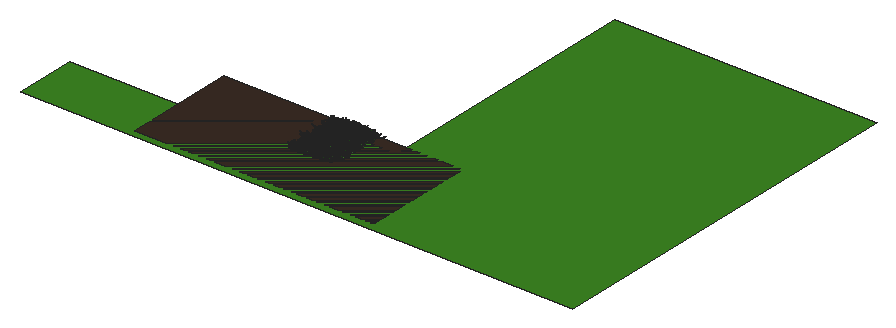
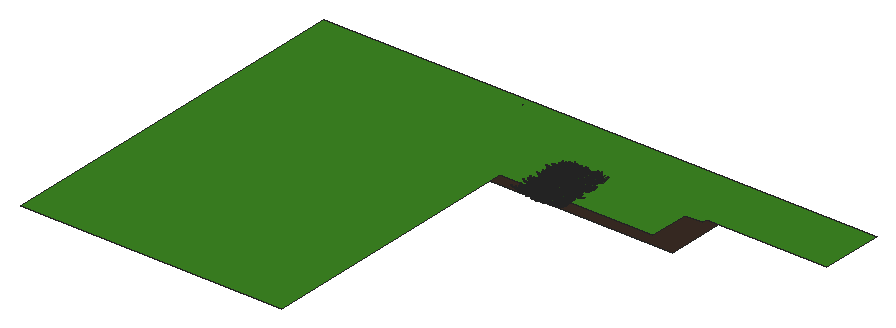
# SketchUp Ruby script. Lengths in inches.
U = 1.inch
M = Sketchup.active_model
def pt(a) = Geom::Point3d.new(a.map { |v| v * U })
def face(e, loops, mat)
  f = e.add_face(loops[0].map { |a| pt(a) })
  loops[1..].each { |l| e.add_face(l.map { |a| pt(a) }).erase! }
  f.material = f.back_material = mat if mat
  f
end
# faces: each face lists its corners as indices into pts; further lists are holes
def faces(e, pts, list, mat = nil) = list.each { |f| face(e, (f[0].is_a?(Array) ? f : [f]).map { |l| l.map { |i| pts[i] } }, mat) }
# xy, xz, yz: faces in a plane at the given z, y or x. An outline is a flat list of corners, or four numbers for a rectangle; further outlines are holes
def ring(l) = l.size == 4 ? [[l[0], l[1]], [l[2], l[1]], [l[2], l[3]], [l[0], l[3]]] : l.each_slice(2).to_a
def flat(e, list, mat, &to3) = list.each { |f| face(e, (f[0].is_a?(Array) ? f : [f]).map { |l| ring(l).map { |u, v| to3.(u, v) } }, mat) }
def xy(e, z, list, mat = nil) = flat(e, list, mat) { |x, y| [x, y, z] }
def xz(e, y, list, mat = nil) = flat(e, list, mat) { |x, z| [x, y, z] }
def yz(e, x, list, mat = nil) = flat(e, list, mat) { |y, z| [x, y, z] }
def lines(e, pts, list) = list.each { |a, b| e.add_line(pt(pts[a]), pt(pts[b])) }
# prism: a flat outline (further loops are holes) pulled along v
def prism(e, loops, v, mat = nil)
  f = face(e, loops, mat); d = Geom::Vector3d.new(v.map { |x| x * U })
  f.pushpull(f.normal.samedirection?(d) ? d.length : -d.length)
end
def box(e, o, s, mat = nil) = prism(e, [[o, [o[0] + s[0], o[1], o[2]], [o[0] + s[0], o[1] + s[1], o[2]], [o[0], o[1] + s[1], o[2]]]], [0, 0, s[2]], mat)
def at(x, y, z, deg = 0) = Geom::Transformation.translation(pt([x, y, z])) * Geom::Transformation.rotation(ORIGIN, Z_AXIS, deg.degrees)
def axes(o, x, y, z) = Geom::Transformation.new([*x, 0, *y, 0, *z, 0, *pt(o).to_a, 1])
def part(name) = M.definitions.add(name)
# library, detail: a bought-in or finely detailed component or shape, given as its bounding box
def library(name, o, s) = part(name).tap { |d| box(d.entities, o, s) }
def detail(e, o, s) = box(e.add_group.entities, o, s)
def put(e, d, t, mat = nil) = e.add_instance(d, t).tap { |i| i.material = mat if mat }
def group(e, t, mat = nil) = e.add_group.tap { |g| g.transformation = t; g.material = mat if mat }.entities
root = M.entities
M.materials.add("Material82").color = [68, 110, 58]
M.materials.add("Material83").color = [48, 90, 38]
M.materials.add("Material84").color = [68, 110, 48]
M.materials.add("Material85").color = [48, 90, 48]
M.materials.add("Material86").color = [58, 110, 58]
M.materials.add("Material87").color = [58, 90, 38]
M.materials.add("Material88").color = [68, 100, 58]
M.materials.add("Material89").color = [48, 100, 38]
M.materials.add("[Color M01]").color = [60, 133, 34]
M.materials.add("top-soil").color = [58, 44, 36]
c1 = part("grass00")
p = [[-0.6875,0.15,0],[-0.56,0.08,5.52],[-0.04,0.03,2.76],[0.48,-0.02,0],[0.35,-0.02,5.52],[-0.1,-0.14,5.52],
  [-0.12,0.65,8.37],[-0.42,0.65,8.37]]
faces(c1.entities,p,[[0,1,2,3],[3,2,4],[1,5,2],[5,4,2],[1,6,5],[4,5,6],[7,6,1]])
c2 = part("Group16\#1")
put(c2.entities,c1,axes([1.44,-0.61,-0.01],[0.05352,0.12609,0],[-0.10704,0.04543,0.07239],[0.06664,-0.02828,0.11628]),"Material85")
put(c2.entities,c1,axes([0.76,-0.15,-0.01],[0.04676,0.24062,0],[-0.23162,0.04501,0.06642],[0.0652,-0.01267,0.23595]),"Material82")
put(c2.entities,c1,axes([0.79,0.01,-0.01],[-0.00606,0.34651,0],[-0.34381,-0.00602,0.0432],[0.04319,0.00076,0.34386]))
put(c2.entities,c1,axes([1,0.23,-0.01],[-0.07192,0.31144,0],[-0.28722,-0.06632,0.1236],[0.12043,0.02781,0.29478]),"Material84")
put(c2.entities,c1,axes([1.66,0.77,-0.01],[-0.13828,0.29651,0],[-0.21551,-0.1005,0.22471],[0.20365,0.09498,0.23779]),"Material89")
put(c2.entities,c1,axes([0.6875,0.52,-0.01],[-0.18126,0.24051,0],[-0.22746,-0.17142,0.09788],[0.07817,0.05891,0.28481]),"Material84")
put(c2.entities,c1,axes([0.68,0.78,-0.01],[-0.215,0.18688,0],[-0.12385,-0.14248,0.21334],[0.13995,0.16101,0.18878]),"Material82")
put(c2.entities,c1,axes([0.56,1,-0.01],[-0.13756,0.07624,0],[-0.06159,-0.11112,0.0927],[0.04494,0.08108,0.12705]),"Material84")
put(c2.entities,c1,axes([0.2,0.64,-0.01],[-0.23729,0.07254,0],[-0.05711,-0.18681,0.153],[0.04473,0.14632,0.19535]),"Material89")
put(c2.entities,c1,axes([0.0625,0.72,-0.01],[-0.28874,0.02525,0],[-0.02179,-0.24916,0.14647],[0.01276,0.14591,0.25012]),"Material82")
put(c2.entities,c1,axes([-0.08,0.62,-0.01],[-0.34089,-0.04187,0],[0.03255,-0.26504,0.216],[-0.02633,0.21439,0.26703]),"Material89")
put(c2.entities,c1,axes([-0.34,0.98,-0.01],[-0.14314,-0.0493,0],[0.04397,-0.12769,0.06843],[-0.02228,0.0647,0.13505]),"Material89")
put(c2.entities,c1,axes([-0.87,1.45,-0.01],[-0.23488,-0.14114,0],[0.13761,-0.22901,0.06087],[-0.03135,0.05217,0.26717]))
put(c2.entities,c1,axes([-0.72,0.77,-0.01],[-0.14208,-0.13251,0],[0.07209,-0.0773,0.16301],[-0.11118,0.11922,0.1057]),"Material89")
put(c2.entities,c1,axes([-0.62,0.43,-0.01],[-0.14845,-0.21203,0],[0.18654,-0.13061,0.12304],[-0.10079,0.07057,0.22772]),"Material82")
put(c2.entities,c1,axes([-0.68,0.29,-0.01],[-0.13639,-0.32136,0],[0.31723,-0.13464,0.05579],[-0.05136,0.0218,0.34462]),"Material83")
put(c2.entities,c1,axes([-0.64,0.125,-0.01],[-0.0458,-0.23569,0],[0.22124,-0.043,0.08276],[-0.08124,0.01579,0.22538]),"Material86")
put(c2.entities,c1,axes([-1.6,-0.03,-0.01],[0.00576,-0.32897,0],[0.27526,0.00482,0.18018],[-0.18015,-0.00315,0.2753]),"Material84")
put(c2.entities,c1,axes([-1.36,-0.31,-0.01],[0.05718,-0.24765,0],[0.18172,0.04196,0.17267],[-0.16825,-0.03885,0.1865]),"Material89")
put(c2.entities,c1,axes([-1.54,-0.72,-0.01],[0.06537,-0.14017,0],[0.13555,0.06321,0.03939],[-0.0357,-0.01665,0.14956]))
put(c2.entities,c1,axes([-1.19,-0.9,-0.01],[0.09597,-0.12735,0],[0.11214,0.08451,0.07557],[-0.06035,-0.04548,0.14042]),"Material88")
put(c2.entities,c1,axes([-0.47,-0.54,-0.01],[0.11588,-0.10072,0],[0.0618,0.0711,0.12124],[-0.07953,-0.0915,0.0942]))
put(c2.entities,c1,axes([-0.47,-0.84,-0.01],[0.11927,-0.0661,0],[0.06603,0.11913,0.00646],[-0.00313,-0.00565,0.13621]),"Material84")
put(c2.entities,c1,axes([-0.38,-1.24,-0.01],[0.28037,-0.08571,0],[0.0618,0.20215,0.20315],[-0.05939,-0.19428,0.21139]),"Material88")
put(c2.entities,c1,axes([-0.06,-0.66,-0.01],[0.22719,-0.01987,0],[0.01247,0.14255,0.17758],[-0.01547,-0.17691,0.1431]),"Material87")
put(c2.entities,c1,axes([0.11,-0.89,-0.01],[0.14882,0.01828,0],[-0.01058,0.08611,0.12229],[0.01491,-0.12138,0.08676]),"Material85")
put(c2.entities,c1,axes([0.25,-0.72,-0.01],[0.20481,0.07053,0],[-0.06206,0.18022,0.10291],[0.03351,-0.0973,0.1906]),"Material85")
put(c2.entities,c1,axes([0.85,-1.42,-0.01],[0.16481,0.09904,0],[-0.09472,0.15762,0.05616],[0.02893,-0.04814,0.18389]),"Material84")
put(c2.entities,c1,axes([1.01,-1.09,-0.01],[0.21858,0.20385,0],[-0.17495,0.1876,0.15339],[0.10462,-0.11218,0.25652]),"Material89")
put(c2.entities,c1,axes([1.01,-0.71,-0.01],[0.08733,0.12473,0],[-0.06445,0.04512,0.13037],[0.1068,-0.07477,0.07867]),"Material85")
c3 = part("Group15\#1")
put(c3.entities,c2,at(0,0,0))
c4 = part("3darcstudiotree_grass00\#1")
put(c4.entities,c3,at(0,0,0))
xy(root,-29.74,[[1534.38,932.5,2096.625,932.5,2096.625,1318.18,1830.75,1318.18,1830.75,1040.81,1674.65,1040.81,1674.65,1000.12,1657.0625,1000.12,1657.0625,994.94,1534.38,994.94]],"[Color M01]")
xy(root,-29.74,[[1644.58,940.12,1887.61,1053.55]],"top-soil")
put(root,c4,axes([1764.68,1016.65,-29.74],[4.10776,0.45174,0],[-0.96091,1.35899,-0.03867],[-0.06802,0.0962,1.75619]))
put(root,c4,axes([1765.02,1044.86,-29.74],[0.30119,1.56993,0],[-3.74927,0.11187,-0.04286],[-0.21599,0.00644,1.42447]))
put(root,c4,axes([1766.64,1014.64,-29.74],[-3.02492,-1.16677,0],[2.80082,-1.12934,-0.0483],[0.17838,-0.07192,1.58573]))
put(root,c4,axes([1765.85,1046.92,-29.74],[3.50639,-1.07574,0],[2.8139,1.42651,-0.05588],[0.16686,0.08459,1.67045]))
put(root,c4,axes([1765.35,996.91,-29.74],[-0.3994,1.69229,0],[-4.36532,-0.16024,-0.02425],[-0.12976,-0.00476,1.76617]))
put(root,c4,axes([1767.22,1050.84,-29.74],[-0.91614,-1.55858,0],[4.47177,-0.40881,-0.01344],[0.0544,-0.00497,1.42931]))
put(root,c4,axes([1766.54,1031.09,-29.74],[-3.80907,0.85988,0],[-1.7501,-1.20575,-0.03218],[-0.10036,-0.06914,1.65786]))
put(root,c4,axes([1767.08,1001.97,-29.74],[1.67083,-1.60234,0],[3.7829,0.6135,-0.00107],[0.00454,0.00074,1.41133]))
put(root,c4,axes([1766.38,1049.21,-29.74],[-1.98309,1.36521,0],[-3.29696,-0.74485,-0.00674],[-0.03007,-0.00679,1.46389]))
put(root,c4,axes([1766.67,1011.9,-29.74],[-1.6341,1.38385,0],[-3.29524,-0.60518,-0.01596],[-0.09907,-0.01819,1.86544]))
put(root,c4,axes([1766.9,1017.96,-29.74],[-1.88391,1.25543,0],[-3.77395,-0.8808,-0.04665],[-0.1806,-0.04215,1.47851]))
put(root,c4,axes([1767.98,1041.09,-29.74],[-3.20908,-0.65771,0],[1.52004,-1.1535,-0.02241],[0.0705,-0.0535,1.68548]))
put(root,c4,axes([1767.1,1030.31,-29.74],[2.49471,1.02577,0],[-2.71621,1.02741,-0.02632],[-0.13149,0.04974,1.95302]))
put(root,c4,axes([1767.45,1037.94,-29.74],[4.09109,-0.59758,0],[1.20224,1.2801,-0.03178],[0.07676,0.08173,1.80429]))
put(root,c4,axes([1767.26,1005.53,-29.74],[2.32026,0.93484,0],[-2.86948,1.10768,-0.01876],[-0.07886,0.03044,1.77063]))
put(root,c4,axes([1767.99,1024.48,-29.74],[0.18236,1.53314,0],[-4.12116,0.07624,-0.04808],[-0.2649,0.0049,1.70557]))
put(root,c4,axes([1767.45,1028.03,-29.74],[1.69594,1.55136,0],[-4.25972,0.72425,-0.01792],[-0.06344,0.01079,1.34035]))
put(root,c4,axes([1770.14,1040.77,-29.74],[-0.92548,-1.44714,0],[3.73119,-0.37112,-0.02503],[0.12441,-0.01237,1.47852]))
put(root,c4,axes([1769.68,1011.59,-29.74],[-3.65717,1.04753,0],[-2.10189,-1.14131,-0.02785],[-0.11272,-0.06121,1.84622]))
put(root,c4,axes([1769.66,1023.08,-29.74],[2.69686,-1.18339,0],[2.47302,0.87653,-0.01288],[0.05957,0.02111,1.54961]))
put(root,c4,axes([1770.53,1016.28,-29.74],[-3.84397,-0.38485,0],[1.07963,-1.67717,-0.00944],[0.01366,-0.02122,1.93444]))
put(root,c4,axes([1770.375,1009.79,-29.74],[-1.0379,-1.53247,0],[3.79206,-0.39944,-0.04991],[0.21721,-0.02288,1.32514]))
put(root,c4,axes([1770.51,1007.98,-29.74],[1.97874,-1.59829,0],[3.60248,0.69366,-0.03421],[0.19371,0.0373,1.89316]))
put(root,c4,axes([1769.73,1025.5625,-29.74],[1.07752,1.49554,0],[-4.17421,0.46775,-0.01918],[-0.10688,0.01198,1.88463]))
put(root,c4,axes([1771.23,1038.75,-29.74],[-3.20067,0.8851,0],[-2.09814,-1.18003,-0.04222],[-0.15558,-0.0875,1.75818]))
put(root,c4,axes([1772.21,1034.17,-29.74],[-3.27374,-0.87824,0],[2.36689,-1.37221,-0.01911],[0.04526,-0.02624,1.32815]))
put(root,c4,axes([1771.875,1005.6,-29.74],[-0.05891,-1.32731,0],[4.1482,-0.02863,-0.04239],[0.194,-0.00134,1.42343]))
put(root,c4,axes([1771.92,1042.43,-29.74],[-3.68407,-0.02356,0],[0.06081,-1.47897,-0.00434],[0.00034,-0.00838,1.37632]))
put(root,c4,axes([1770.62,1051.3,-29.74],[3.58378,0.39823,0],[-1.22974,1.72119,-0.04858],[-0.06101,0.08539,1.57379]))
put(root,c4,axes([1772.68,1021.25,-29.74],[-0.12973,-1.5282,0],[4.23676,-0.05594,-0.02714],[0.12341,-0.00163,1.44559]))
put(root,c4,axes([1772.24,1030.24,-29.74],[-3.75575,0.69708,0],[-1.71963,-1.441,-0.0027],[-0.006,-0.00502,1.57765]))
put(root,c4,axes([1772.29,1049.52,-29.74],[-2.752,0.72492,0],[-2.08218,-1.22939,-0.04884],[-0.13401,-0.07912,1.38796]))
put(root,c4,axes([1772.3,999.63,-29.74],[2.6038,-1.3441,0],[3.00735,0.90609,-0.00592],[0.02965,0.00893,1.78738]))
put(root,c4,axes([1773.15,1000.67,-29.74],[-2.61082,-1.14432,0],[2.90627,-1.03127,-0.02928],[0.10098,-0.03583,1.35967]))
put(root,c4,axes([1773.4,1046.52,-29.74],[-3.67064,-0.9709,0],[1.88491,-1.10833,-0.03319],[0.11926,-0.07012,1.63594]))
put(root,c4,axes([1772.1,1035.62,-29.74],[-0.84248,1.5623,0],[-4.12413,-0.34589,-0.02719],[-0.15102,-0.01267,1.79436]))
put(root,c4,axes([1772.375,1026.67,-29.74],[-0.14307,1.431,0],[-4.32963,-0.06732,-0.01193],[-0.07261,-0.00113,1.97773]))
put(root,c4,axes([1773.25,1032.0625,-29.74],[-0.69376,1.57067,0],[-3.29157,-0.22612,-0.03897],[-0.27242,-0.01871,1.77692]))
put(root,c4,axes([1773.14,1014.9,-29.74],[-0.09674,1.30199,0],[-3.40883,-0.03939,-0.04664],[-0.25839,-0.00299,1.41669]))
put(root,c4,axes([1772.72,997.3125,-29.74],[0.99401,1.39114,0],[-3.81883,0.42439,-0.02067],[-0.11338,0.0126,1.69495]))
put(root,c4,axes([1773.09,1019.4375,-29.74],[2.79143,1.2628,0],[-2.51561,0.86486,-0.0286],[-0.15611,0.05367,1.81122]))
put(root,c4,axes([1773.33,1003.83,-29.74],[-0.55757,1.6642,0],[-4.56304,-0.23777,-0.03274],[-0.13576,-0.00707,1.44297]))
put(root,c4,axes([1773.17,1044.85,-29.74],[3.6798,1.00569,0],[-2.52504,1.43694,-0.01195],[-0.02817,0.01603,1.37528]))
put(root,c4,axes([1775.23,1034,-29.74],[-4.22095,0.29279,0],[-0.61258,-1.3735,-0.03096],[-0.02808,-0.06297,1.38775]))
put(root,c4,axes([1775.42,1018.77,-29.74],[-3.21861,0.39731,0],[-1.33805,-1.68585,-0.0251],[-0.03563,-0.04489,1.59541]))
put(root,c4,axes([1775.95,1049.15,-29.74],[-3.05504,-0.78096,0],[2.06441,-1.25601,-0.04254],[0.14556,-0.08856,1.78955]))
put(root,c4,axes([1775.45,1031.19,-29.74],[-2.75394,0.84395,0],[-2.86283,-1.45294,-0.03993],[-0.13572,-0.06888,1.9372]))
put(root,c4,axes([1776.33,1037.82,-29.74],[-4.11616,0.08361,0],[-0.21641,-1.65704,-0.00589],[-0.00131,-0.01,1.35922]))
put(root,c4,axes([1775.47,1005.03,-29.74],[0.77539,1.49335,0],[-4.15697,0.3357,-0.02758],[-0.13791,0.01114,1.62317]))
put(root,c4,axes([1777.24,1051.72,-29.74],[0.31357,-1.68647,0],[3.44554,0.09964,-0.00239],[0.01314,0.00038,1.42634]))
put(root,c4,axes([1775.74,1020.25,-29.74],[0.83918,1.59477,0],[-3.76377,0.30803,-0.00381],[-0.02098,0.00172,1.62105]))
put(root,c4,axes([1777.45,1042.99,-29.74],[-4.10797,-0.04724,0],[0.09871,-1.33508,-0.0193],[0.00442,-0.0598,1.99558]))
put(root,c4,axes([1777.5,1013.81,-29.74],[-4.69627,0.21945,0],[-0.46002,-1.53114,-0.03012],[-0.01578,-0.05252,1.30483]))
put(root,c4,axes([1776.42,1001,-29.74],[-1.57534,1.27293,0],[-3.92925,-0.75629,-0.02753],[-0.13899,-0.02675,1.84121]))
put(root,c4,axes([1776.8,1003.97,-29.74],[2.05797,-1.09603,0],[2.87826,0.84054,-0.04843],[0.25021,0.07307,1.72564]))
put(root,c4,axes([1777.49,1046.3125,-29.74],[0.58086,-1.47611,0],[3.37891,0.2068,-0.00401],[0.02817,0.00172,1.82024]))
put(root,c4,axes([1777.82,1023.3,-29.74],[1.23956,-1.20185,0],[3.42028,0.54865,-0.0011],[0.00669,0.00107,1.80895]))
put(root,c4,axes([1777.88,1011.9375,-29.74],[0.89327,-1.81074,0],[4.0321,0.30937,-0.02432],[0.12035,0.00923,1.55217]))
put(root,c4,axes([1778.76,1009.77,-29.74],[0.20119,-1.37174,0],[3.84475,0.0877,-0.03098],[0.16829,0.00384,1.57088]))
put(root,c4,axes([1779.24,1027.92,-29.74],[-3.63168,-0.94551,0],[2.04917,-1.22414,-0.0411],[0.11661,-0.06966,1.43569]))
put(root,c4,axes([1779.11,1008.55,-29.74],[-0.37192,-1.4591,0],[3.79295,-0.15037,-0.02999],[0.19954,-0.00791,1.91089]))
put(root,c4,axes([1778.84,1024.8,-29.74],[2.01038,-1.40201,0],[3.67214,0.81896,-0.04614],[0.18867,0.04208,1.48544]))
put(root,c4,axes([1778.87,998.42,-29.74],[3.21693,-1.31198,0],[2.89205,1.10289,-0.03201],[0.144,0.05492,1.88682]))
put(root,c4,axes([1778.42,1041.03,-29.74],[4.09331,0.01199,0],[-0.0289,1.53398,-0.04293],[-0.00148,0.07869,1.35522]))
put(root,c4,axes([1778.89,1028.8125,-29.74],[3.51633,-0.36112,0],[0.9428,1.4278,-0.03218],[0.03818,0.05783,1.32043]))
put(root,c4,axes([1779.11,1036.08,-29.74],[3.55776,-0.23199,0],[0.75341,1.79699,-0.01648],[0.0118,0.02815,1.51991]))
put(root,c4,axes([1779.24,1045.42,-29.74],[-0.04316,1.58062,0],[-4.72981,-0.02009,-0.05791],[-0.26281,-0.00112,1.60897]))
put(root,c4,axes([1779.08,1015.79,-29.74],[4.6177,0.37892,0],[-0.96466,1.82835,-0.01168],[-0.00936,0.01774,1.39591]))
put(root,c4,axes([1781.29,998.21,-29.74],[2.466,-1.02389,0],[3.09141,1.158,-0.03691],[0.15975,0.05984,1.90749]))
put(root,c4,axes([1782.25,1021.22,-29.74],[-2.89327,-0.98526,0],[2.3422,-1.06973,-0.01919],[0.0931,-0.04252,1.99409]))
put(root,c4,axes([1780.64,1051.875,-29.74],[4.65922,-0.05932,0],[0.11762,1.43686,-0.01793],[0.0038,0.04639,1.79317]))
put(root,c4,axes([1782.5,1006.3125,-29.74],[-3.01308,-1.39849,0],[3.33443,-1.11734,-0.06095],[0.24941,-0.08358,1.76096]))
put(root,c4,axes([1782.34,1043.12,-29.74],[0.00434,-1.45328,0],[3.77222,0.00175,-0.01884],[0.09694,0.00004,1.45492]))
put(root,c4,axes([1782.34,1010.48,-29.74],[1.17396,-1.50467,0],[4.45897,0.54108,-0.02541],[0.10297,0.01249,1.48254]))
put(root,c4,axes([1782.32,1044.97,-29.74],[-3.66261,0.69653,0],[-1.57298,-1.28643,-0.02015],[-0.06083,-0.04975,1.88684]))
put(root,c4,axes([1783.04,1016.42,-29.74],[-3.89542,-0.50736,0],[1.22292,-1.46031,-0.04962],[0.09609,-0.11475,1.8049]))
put(root,c4,axes([1782.42,1008.33,-29.74],[-2.84312,0.65512,0],[-2.18872,-1.47733,-0.05376],[-0.11522,-0.07777,1.38154]))
put(root,c4,axes([1781.92,1019.12,-29.74],[-0.91872,1.71096,0],[-4.38194,-0.36595,-0.05285],[-0.26515,-0.02214,1.72177]))
put(root,c4,axes([1783.39,1053.02,-29.74],[-1.59587,-1.14266,0],[4.12201,-0.89537,-0.06742],[0.26463,-0.05748,1.58058]))
put(root,c4,axes([1782.68,1027.27,-29.74],[-2.79487,1.34009,0],[-3.4856,-1.13062,-0.01702],[-0.07434,-0.02411,1.91367]))
put(root,c4,axes([1782.47,1048.65,-29.74],[4.14299,-0.56741,0],[1.47163,1.6712,-0.03586],[0.0631,0.07166,1.80381]))
put(root,c4,axes([1782.65,1001.45,-29.74],[4.14821,-0.06928,0],[0.17152,1.59736,-0.02002],[0.00473,0.044,1.69539]))
put(root,c4,axes([1783.96,1038.57,-29.74],[-4.14933,0.35699,0],[-0.86081,-1.55612,-0.03649],[-0.04634,-0.08377,1.80375]))
put(root,c4,axes([1782.63,1033.55,-29.74],[4.28763,0.74332,0],[-1.60811,1.44267,-0.02572],[-0.05083,0.0456,1.47108]))
put(root,c4,axes([1784.51,1013.68,-29.74],[-3.82686,-0.23596,0],[0.71117,-1.79387,-0.04342],[0.03245,-0.08186,1.66984]))
put(root,c4,axes([1783.4375,1024.92,-29.74],[-1.95951,1.68141,0],[-3.84767,-0.6974,-0.02861],[-0.15441,-0.02799,1.88512]))
put(root,c4,axes([1784.35,1030.23,-29.74],[-0.85342,-1.31702,0],[3.52172,-0.35493,-0.03508],[0.23842,-0.02403,1.91126]))
put(root,c4,axes([1784.5625,1011.45,-29.74],[-3.45153,-0.0864,0],[0.28769,-1.78743,-0.04372],[0.01068,-0.06634,1.31241]))
put(root,c4,axes([1784.14,1032.29,-29.74],[-1.89755,1.14164,0],[-2.79539,-0.72263,-0.04],[-0.1948,-0.05036,1.45882]))
put(root,c4,axes([1784.7,1040.67,-29.74],[-4.56188,0.50767,0],[-1.2186,-1.7031,-0.00145],[-0.00214,-0.00299,1.8291]))
put(root,c4,axes([1783.59,1047.56,-29.74],[-0.0946,1.80399,0],[-4.6355,-0.03781,-0.04199],[-0.20347,-0.00166,1.68448]))
put(root,c4,axes([1783.84,1035.81,-29.74],[3.68176,-0.08889,0],[0.28452,1.83295,-0.0507],[0.01477,0.09515,1.66388]))
put(root,c4,axes([1783.96,1022.99,-29.74],[1.28845,1.74913,0],[-3.19455,0.36599,-0.00931],[-0.04886,0.0056,1.3628]))
put(root,c4,axes([1784.73,1004.1,-29.74],[3.2366,-0.57131,0],[1.58048,1.39258,-0.04939],[0.12568,0.11074,1.80606]))
put(root,c4,axes([1786.37,1032.03,-29.74],[-3.02696,1.26281,0],[-2.89442,-1.07905,-0.01805],[-0.07526,-0.02806,1.71251]))
put(root,c4,axes([1786.83,1025.5,-29.74],[-3.18632,0.63668,0],[-1.6075,-1.25121,-0.00642],[-0.0144,-0.01121,1.3229]))
put(root,c4,axes([1787.45,1001.04,-29.74],[-3.56938,-0.43544,0],[1.36231,-1.73682,-0.06046],[0.07694,-0.09809,1.48798]))
put(root,c4,axes([1786.67,1035.32,-29.74],[-2.26269,0.97698,0],[-3.46591,-1.24844,-0.00484],[-0.01583,-0.0057,1.55938]))
put(root,c4,axes([1786.99,998.84,-29.74],[-3.08205,1.07293,0],[-3.11637,-1.39229,-0.01862],[-0.0666,-0.02976,1.90809]))
put(root,c4,axes([1788.17,1029.41,-29.74],[-1.06768,-1.28552,0],[4.42505,-0.5716,-0.01545],[0.0652,-0.00842,1.54954]))
put(root,c4,axes([1788.23,997.44,-29.74],[-0.50603,-1.39331,0],[4.58553,-0.25902,-0.00214],[0.00976,-0.00055,1.59988]))
put(root,c4,axes([1786.96,1016.83,-29.74],[-2.17882,1.11223,0],[-3.27984,-0.99929,-0.01374],[-0.05934,-0.01808,1.69563]))
put(root,c4,axes([1786.625,1005.88,-29.74],[-1.12838,1.66356,0],[-4.06225,-0.42855,-0.00132],[-0.00752,-0.00079,1.858]))
put(root,c4,axes([1786.24,1023.17,-29.74],[3.24771,1.22669,0],[-3.17033,1.30544,-0.01961],[-0.06543,0.02694,1.65716]))
put(root,c4,axes([1788.08,1003.25,-29.74],[-3.65901,0.17551,0],[-0.56536,-1.83311,-0.00408],[-0.00246,-0.00797,1.74968]))
put(root,c4,axes([1786.67,1045.58,-29.74],[0.64791,1.78613,0],[-4.32576,0.24405,-0.02596],[-0.10407,0.00587,1.32635]))
put(root,c4,axes([1786.88,1026.68,-29.74],[-1.07809,1.72568,0],[-4.31745,-0.4195,-0.00818],[-0.04348,-0.00422,1.82396]))
put(root,c4,axes([1787.1875,1047.25,-29.74],[2.43664,1.45627,0],[-2.82206,0.73439,-0.04277],[-0.22349,0.05816,1.58679]))
put(root,c4,axes([1787.84,1038.88,-29.74],[4.1241,0.10126,0],[-0.23149,1.46627,-0.04181],[-0.01816,0.11501,1.95138]))
put(root,c4,axes([1789.07,1050.66,-29.74],[-3.5428,1.01388,0],[-2.21614,-1.2044,-0.01293],[-0.05166,-0.02807,1.92389]))
put(root,c4,axes([1787.8125,1020.17,-29.74],[2.96136,1.19987,0],[-3.11013,1.19384,-0.004],[-0.01667,0.0064,1.89371]))
put(root,c4,axes([1789.61,1010.4375,-29.74],[-4.14748,0.25836,0],[-0.59761,-1.49206,-0.01239],[-0.00958,-0.02393,1.42361]))
put(root,c4,axes([1788.36,1007.84,-29.74],[4.21182,0.14848,0],[-0.32581,1.4374,-0.01038],[-0.00654,0.02884,1.94021]))
put(root,c4,axes([1788.37,1033.9,-29.74],[4.10391,0.70985,0],[-1.57565,1.41679,-0.04488],[-0.12117,0.10895,1.97665]))
put(root,c4,axes([1788.49,1012.47,-29.74],[1.10995,1.51966,0],[-3.58981,0.40779,-0.02733],[-0.15418,0.01751,1.64375]))
put(root,c4,axes([1789.53,1048.79,-29.74],[2.20641,-0.98098,0],[3.35125,1.17232,-0.037],[0.12603,0.04409,1.52862]))
put(root,c4,axes([1789.42,1042.75,-29.74],[2.40726,1.00896,0],[-2.45133,0.90962,-0.04643],[-0.23456,0.08704,1.7498]))
put(root,c4,axes([1789.42,1040.88,-29.74],[1.86032,1.34861,0],[-2.96544,0.63621,-0.01685],[-0.11323,0.02429,1.93576]))
put(root,c4,axes([1789.67,1019.48,-29.74],[4.19014,0.72772,0],[-1.46084,1.30821,-0.04159],[-0.08773,0.07856,1.42181]))
put(root,c4,axes([1791.72,1007.11,-29.74],[-1.84068,-1.59832,0],[3.91902,-0.70195,-0.02239],[0.11993,-0.02148,1.89813]))
put(root,c4,axes([1790.24,1013.75,-29.74],[0.99879,1.74855,0],[-3.87665,0.3444,-0.04632],[-0.24296,0.02158,1.6013]))
put(root,c4,axes([1792.18,1036.375,-29.74],[-4.27172,-0.34301,0],[0.88739,-1.71879,-0.03896],[0.04123,-0.07985,1.76791]))
put(root,c4,axes([1791.86,1034.52,-29.74],[3.05285,-0.84724,0],[2.57962,1.44566,-0.04926],[0.16288,0.09128,1.93034]))
put(root,c4,axes([1792.16,1040.04,-29.74],[-2.93173,0.8474,0],[-2.63832,-1.41962,-0.02359],[-0.06961,-0.03745,1.66971]))
put(root,c4,axes([1793.22,1050.04,-29.74],[-4.04158,-0.94067,0],[1.75814,-1.17484,-0.01139],[0.03404,-0.02275,1.52439]))
put(root,c4,axes([1793.33,1000.93,-29.74],[-0.45548,-1.68091,0],[3.45741,-0.14571,-0.01446],[0.0889,-0.00375,1.61179]))
put(root,c4,axes([1792.78,999.58,-29.74],[-3.13157,0.80525,0],[-2.19448,-1.32731,-0.02083],[-0.06068,-0.0367,1.60618]))
put(root,c4,axes([1793.68,1046.52,-29.74],[-3.80321,-0.44648,0],[1.10938,-1.46975,-0.0137],[0.0187,-0.02478,1.39479]))
put(root,c4,axes([1794.04,1020.97,-29.74],[-3.37995,-1.26993,0],[3.24999,-1.34532,-0.03405],[0.09733,-0.04029,1.46358]))
put(root,c4,axes([1792.0625,1012.8125,-29.74],[1.40547,1.51439,0],[-4.0139,0.57938,-0.03042],[-0.14333,0.02069,1.60735]))
put(root,c4,axes([1792.49,1027.1875,-29.74],[4.00543,0.63259,0],[-1.51384,1.49079,-0.05201],[-0.11143,0.10973,1.75905]))
put(root,c4,axes([1793.46,1044.91,-29.74],[3.22644,-0.51746,0],[1.32565,1.28555,-0.02601],[0.05462,0.05297,1.4702]))
put(root,c4,axes([1793.21,1038.28,-29.74],[4.21739,-0.2744,0],[0.59088,1.41243,-0.03976],[0.04192,0.1002,1.7619]))
put(root,c4,axes([1793.68,1005.62,-29.74],[-0.09951,1.54184,0],[-3.8951,-0.0391,-0.03168],[-0.18001,-0.00181,1.66016]))
put(root,c4,axes([1794.22,1023.28,-29.74],[3.13004,-0.71111,0],[2.12935,1.45771,-0.00508],[0.01244,0.00852,1.56982]))
put(root,c4,axes([1793.78,1018.96,-29.74],[1.71903,1.73474,0],[-3.69921,0.57012,-0.05423],[-0.23247,0.03583,1.37014]))
put(root,c4,axes([1795.21,1014.42,-29.74],[1.52517,-1.72025,0],[3.68343,0.50792,-0.01723],[0.07984,0.01101,1.43549]))
put(root,c4,axes([1794.76,1003.85,-29.74],[-2.42659,1.57566,0],[-3.75552,-0.89953,-0.06137],[-0.23264,-0.05572,1.46064]))
put(root,c4,axes([1794.44,1009.48,-29.74],[3.59244,-0.46408,0],[1.16578,1.40355,-0.03684],[0.0661,0.07959,1.61813]))
put(root,c4,axes([1794.66,1051.23,-29.74],[4.25801,-0.4781,0],[1.08249,1.49942,-0.0361],[0.05003,0.0693,1.4995]))
put(root,c4,axes([1795.59,1015.99,-29.74],[-3.02925,1.34013,0],[-2.7234,-0.95744,-0.02096],[-0.09613,-0.0338,1.6805]))
put(root,c4,axes([1795.45,1031.13,-29.74],[-1.53161,1.39817,0],[-3.93212,-0.66992,-0.05011],[-0.24211,-0.04125,1.6899]))
